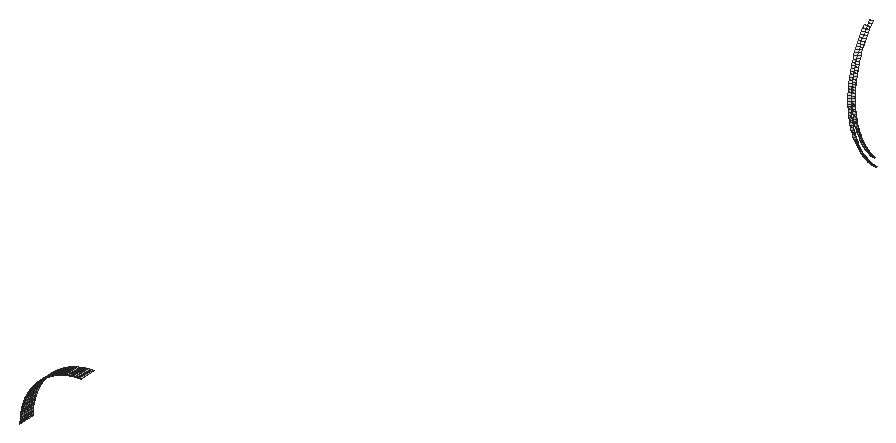
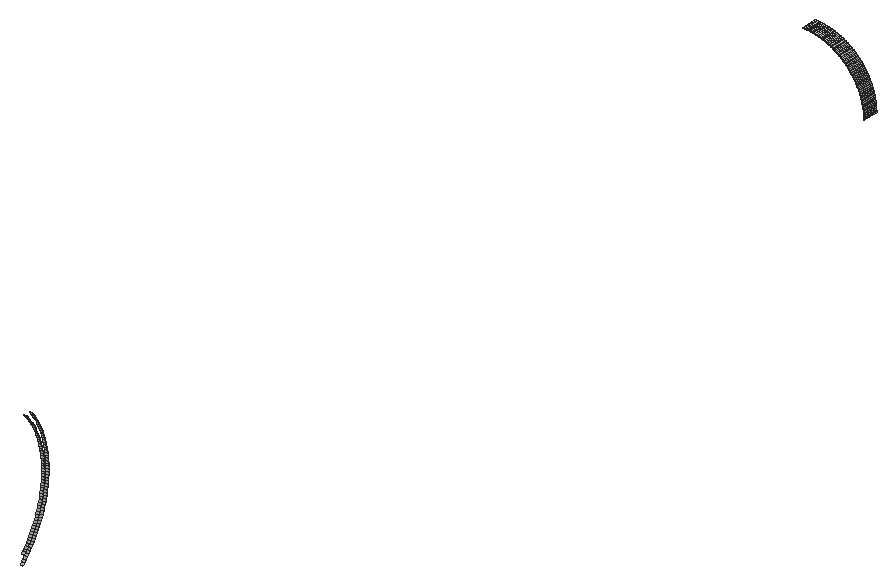
# SketchUp Ruby script. Lengths in inches.
U = 1.inch
M = Sketchup.active_model
def pt(a) = Geom::Point3d.new(a.map { |v| v * U })
def face(e, loops, mat)
  f = e.add_face(loops[0].map { |a| pt(a) })
  loops[1..].each { |l| e.add_face(l.map { |a| pt(a) }).erase! }
  f.material = f.back_material = mat if mat
  f
end
# faces: each face lists its corners as indices into pts; further lists are holes
def faces(e, pts, list, mat = nil) = list.each { |f| face(e, (f[0].is_a?(Array) ? f : [f]).map { |l| l.map { |i| pts[i] } }, mat) }
# xy, xz, yz: faces in a plane at the given z, y or x. An outline is a flat list of corners, or four numbers for a rectangle; further outlines are holes
def ring(l) = l.size == 4 ? [[l[0], l[1]], [l[2], l[1]], [l[2], l[3]], [l[0], l[3]]] : l.each_slice(2).to_a
def flat(e, list, mat, &to3) = list.each { |f| face(e, (f[0].is_a?(Array) ? f : [f]).map { |l| ring(l).map { |u, v| to3.(u, v) } }, mat) }
def xy(e, z, list, mat = nil) = flat(e, list, mat) { |x, y| [x, y, z] }
def xz(e, y, list, mat = nil) = flat(e, list, mat) { |x, z| [x, y, z] }
def yz(e, x, list, mat = nil) = flat(e, list, mat) { |y, z| [x, y, z] }
def lines(e, pts, list) = list.each { |a, b| e.add_line(pt(pts[a]), pt(pts[b])) }
# prism: a flat outline (further loops are holes) pulled along v
def prism(e, loops, v, mat = nil)
  f = face(e, loops, mat); d = Geom::Vector3d.new(v.map { |x| x * U })
  f.pushpull(f.normal.samedirection?(d) ? d.length : -d.length)
end
def box(e, o, s, mat = nil) = prism(e, [[o, [o[0] + s[0], o[1], o[2]], [o[0] + s[0], o[1] + s[1], o[2]], [o[0], o[1] + s[1], o[2]]]], [0, 0, s[2]], mat)
def at(x, y, z, deg = 0) = Geom::Transformation.translation(pt([x, y, z])) * Geom::Transformation.rotation(ORIGIN, Z_AXIS, deg.degrees)
def axes(o, x, y, z) = Geom::Transformation.new([*x, 0, *y, 0, *z, 0, *pt(o).to_a, 1])
def part(name) = M.definitions.add(name)
# library, detail: a bought-in or finely detailed component or shape, given as its bounding box
def library(name, o, s) = part(name).tap { |d| box(d.entities, o, s) }
def detail(e, o, s) = box(e.add_group.entities, o, s)
def put(e, d, t, mat = nil) = e.add_instance(d, t).tap { |i| i.material = mat if mat }
def group(e, t, mat = nil) = e.add_group.tap { |g| g.transformation = t; g.material = mat if mat }.entities
root = M.entities
M.materials.add("[Quartz Light Grey]").color = [251, 251, 252]
xy(root,66,[[23.6875,50,23.84,53],[23.84,50,24,53]])
xz(root,211,[[44.5,50.56,45,51.0625]],"[Quartz Light Grey]")
xz(root,212,[[44.5,50.59,45,51.06]],"[Quartz Light Grey]")
yz(root,12,[[50,54,53,54.16],[50,54.16,53,54.3125]])
p = [[45,216.875,37.26],[45,217.24,36.92],[44.5,217.24,36.92],[44.5,216.875,37.26],[45,216.52,37.61],[44.5,216.52,37.61],
  [45,216.18,37.97],[44.5,216.18,37.97],[45,215.84,38.33],[44.5,215.84,38.33],[45,215.51,38.71],[44.5,215.51,38.71],
  [45,215.2,39.09],[44.5,215.2,39.09],[45,216.9,38.65],[45,216.58,39],[44.5,216.58,39],[44.5,216.9,38.65],
  [45,216.27,39.35],[44.5,216.27,39.35],[45,214.89,39.48],[44.5,214.89,39.48],[45,215.97,39.72],[44.5,215.97,39.72],
  [45,214.59,39.88],[44.5,214.59,39.88],[45,215.68,40.09],[44.5,215.68,40.09],[45,214.31,40.29],[44.5,214.31,40.29],
  [45,215.4,40.47],[44.5,215.4,40.47],[45,214.03,40.7],[44.5,214.03,40.7],[45,215.13,40.85],[44.5,215.13,40.85],
  [45,213.77,41.125],[44.5,213.77,41.125],[45,214.87,41.25],[44.5,214.87,41.25],[45,213.51,41.55],[44.5,213.51,41.55],
  [45,214.62,41.65],[44.5,214.62,41.65],[45,213.27,41.99],[44.5,213.27,41.99],[45,214.38,42.05],[44.5,214.38,42.05],
  [45,213.04,42.43],[44.5,213.04,42.43],[45,214.15,42.46],[44.5,214.15,42.46],[45,212.82,42.875],[44.5,212.82,42.875],
  [45,213.94,42.88],[44.5,213.94,42.88],[45,212.62,43.33],[44.5,212.62,43.33],[45,213.73,43.3],[44.5,213.73,43.3],
  [45,212.42,43.79],[44.5,212.42,43.79],[45,213.53,43.73],[44.5,213.53,43.73],[45,213.35,44.17],[44.5,213.35,44.17],
  [45,212.24,44.25],[44.5,212.24,44.25],[45,212.07,44.72],[44.5,212.07,44.72],[45,213.17,44.6],[44.5,213.17,44.6],
  [45,213.01,45.05],[44.5,213.01,45.05],[45,211.91,45.1875],[44.5,211.91,45.1875],[45,212.86,45.49],[44.5,212.86,45.49],
  [45,211.76,45.66],[44.5,211.76,45.66],[45,212.72,45.94],[44.5,212.72,45.94],[45,211.63,46.14],[44.5,211.63,46.14],
  [45,212.6,46.4],[44.5,212.6,46.4],[45,211.51,46.625],[44.5,211.51,46.625],[45,212.48,46.86],[44.5,212.48,46.86],
  [45,211.4,47.11],[44.5,211.4,47.11],[45,212.38,47.31],[44.5,212.38,47.31],[45,211.31,47.6],[44.5,211.31,47.6],
  [45,212.29,47.78],[44.5,212.29,47.78],[45,211.22,48.09],[44.5,211.22,48.09],[45,212.21,48.24],[44.5,212.21,48.24],
  [45,211.15,48.58],[44.5,211.15,48.58],[45,212.15,48.71],[44.5,212.15,48.71],[45,211.1,49.08],[44.5,211.1,49.08],
  [45,212.09,49.18],[44.5,212.09,49.18],[45,211.05,49.57],[44.5,211.05,49.57],[45,212.05,49.65],[44.5,212.05,49.65],
  [45,211.02,50.07],[44.5,211.02,50.07],[45,212.02,50.12],[44.5,212.02,50.12],[45,211,50.56],[44.5,211,50.56],
  [45,212,50.59],[44.5,212,50.59],[45,211.01,51.56],[45,211,51.0625],[44.5,211,51.0625],[44.5,211.01,51.56],
  [45,212,51.06],[45,212.01,51.53],[44.5,212.01,51.53],[44.5,212,51.06],[45,212.03,52],[44.5,212.03,52],
  [45,211.03,52.06],[44.5,211.03,52.06],[45,212.06,52.47],[44.5,212.06,52.47],[45,211.0625,52.55],[44.5,211.0625,52.55],
  [45,212.1,52.94],[44.5,212.1,52.94],[45,211.11,53.05],[44.5,211.11,53.05],[45,212.16,53.41],[44.5,212.16,53.41],
  [45,211.17,53.54],[44.5,211.17,53.54],[45,212.23,53.875],[44.5,212.23,53.875],[45,211.24,54.03],[44.5,211.24,54.03],
  [45,212.3125,54.34],[44.5,212.3125,54.34],[45,211.33,54.52],[44.5,211.33,54.52],[12,53,54.3125],[12.01,53,54.47],
  [12.01,50,54.47],[12,50,54.3125],[45,212.41,54.8],[44.5,212.41,54.8],[12.02,53,54.63],[12.02,50,54.63],
  [45,211.43,55.01],[44.5,211.43,55.01],[12.03,53,54.78],[12.03,50,54.78],[12.04,53,54.94],[12.04,50,54.94],
  [45,212.51,55.26],[44.5,212.51,55.26],[12.05,53,55.1],[12.05,50,55.1],[45,211.54,55.5],[44.5,211.54,55.5],
  [12.07,53,55.25],[12.07,50,55.25],[12.08,53,55.41],[12.08,50,55.41],[45,212.63,55.72],[44.5,212.63,55.72],
  [12.1,53,55.57],[12.1,50,55.57],[45,211.66,55.98],[44.5,211.66,55.98],[12.125,53,55.72],[12.125,50,55.72],
  [12.15,53,55.88],[12.15,50,55.88],[45,212.76,56.17],[44.5,212.76,56.17],[12.17,53,56.03],[12.17,50,56.03],
  [12.2,53,56.1875],[12.2,50,56.1875],[45,211.8,56.46],[44.5,211.8,56.46],[12.23,53,56.34],[12.23,50,56.34],
  [45,212.9,56.62],[44.5,212.9,56.62],[12.26,53,56.49],[12.26,50,56.49],[12.3,53,56.65],[12.3,50,56.65],
  [45,211.95,56.93],[44.5,211.95,56.93],[12.33,53,56.8],[12.33,50,56.8],[45,213.05,57.0625],[44.5,213.05,57.0625],
  [12.37,53,56.95],[12.37,50,56.95],[45,212.11,57.4],[44.5,212.11,57.4],[12.41,53,57.11],[12.41,50,57.11],
  [12.45,53,57.26],[12.45,50,57.26],[45,213.22,57.51],[44.5,213.22,57.51],[12.49,53,57.41],[12.49,50,57.41],
  [12.54,53,57.56],[12.54,50,57.56],[45,212.28,57.87],[44.5,212.28,57.87],[45,213.39,57.94],[44.5,213.39,57.94],
  [12.59,53,57.71],[12.59,50,57.71],[12.64,53,57.86],[12.64,50,57.86],[12.6875,53,58.01],[12.6875,50,58.01],
  [45,212.47,58.33],[44.5,212.47,58.33],[45,213.58,58.375],[44.5,213.58,58.375],[12.74,53,58.15],[12.74,50,58.15],
  [12.8,53,58.3],[12.8,50,58.3],[12.85,53,58.45],[12.85,50,58.45],[45,212.67,58.78],[44.5,212.67,58.78],
  [12.91,53,58.59],[12.91,50,58.59],[45,213.78,58.8],[44.5,213.78,58.8],[12.97,53,58.74],[12.97,50,58.74],
  [13.04,53,58.88],[13.04,50,58.88],[45,212.88,59.24],[44.5,212.88,59.24],[45,213.99,59.22],[44.5,213.99,59.22],
  [13.1,53,59.02],[13.1,50,59.02],[13.17,53,59.17],[13.17,50,59.17],[13.24,53,59.31],[13.24,50,59.31],
  [45,213.1,59.68],[44.5,213.1,59.68],[45,214.21,59.64],[44.5,214.21,59.64],[13.31,53,59.45],[13.31,50,59.45],
  [13.38,53,59.59],[13.38,50,59.59],[13.45,53,59.73],[13.45,50,59.73],[45,214.44,60.05],[44.5,214.44,60.05],
  [13.53,53,59.86],[13.53,50,59.86],[45,213.33,60.12],[44.5,213.33,60.12],[13.61,53,60],[13.61,50,60],
  [13.6875,53,60.14],[13.6875,50,60.14],[13.77,53,60.27],[13.77,50,60.27],[45,213.58,60.55],[44.5,213.58,60.55],
  [45,214.68,60.45],[44.5,214.68,60.45],[13.85,53,60.4],[13.85,50,60.4],[13.9375,53,60.54],[13.9375,50,60.54],
  [14.02,53,60.67],[14.02,50,60.67],[45,214.9375,60.85],[44.5,214.9375,60.85],[45,213.83,60.98],[44.5,213.83,60.98],
  [14.11,53,60.8],[14.11,50,60.8],[14.2,53,60.93],[14.2,50,60.93],[14.29,53,61.05],[14.29,50,61.05],
  [45,215.2,61.24],[44.5,215.2,61.24],[45,214.1,61.4],[44.5,214.1,61.4],[14.38,53,61.18],[14.38,50,61.18],
  [14.48,53,61.31],[14.48,50,61.31],[45,215.47,61.63],[44.5,215.47,61.63],[14.58,53,61.43],[14.58,50,61.43],
  [14.67,53,61.55],[14.67,50,61.55],[45,214.375,61.8125],[44.5,214.375,61.8125],[14.77,53,61.67],[14.77,50,61.67],
  [45,215.76,62],[44.5,215.76,62],[14.875,53,61.79],[14.875,50,61.79],[14.98,53,61.91],[14.98,50,61.91],
  [45,214.67,62.22],[44.5,214.67,62.22],[15.08,53,62.03],[15.08,50,62.03],[15.1875,53,62.15],[15.1875,50,62.15],
  [45,216.05,62.375],[44.5,216.05,62.375],[15.3,53,62.26],[15.3,50,62.26],[45,214.96,62.62],[44.5,214.96,62.62],
  [15.4,53,62.375],[15.4,50,62.375],[15.51,53,62.49],[15.51,50,62.49],[45,216.35,62.73],[44.5,216.35,62.73],
  [15.625,53,62.6],[15.625,50,62.6],[15.74,53,62.7],[15.74,50,62.7],[15.85,53,62.8125],[15.85,50,62.8125],
  [15.97,53,62.92],[15.97,50,62.92],[16.09,53,63.02],[16.09,50,63.02],[16.21,53,63.125],[16.21,50,63.125],
  [16.33,53,63.23],[16.33,50,63.23],[16.45,53,63.33],[16.45,50,63.33],[16.57,53,63.42],[16.57,50,63.42],
  [16.69,53,63.52],[16.69,50,63.52],[16.82,53,63.62],[16.82,50,63.62],[16.95,53,63.71],[16.95,50,63.71],
  [17.07,53,63.8],[17.07,50,63.8],[17.2,53,63.89],[17.2,50,63.89],[17.33,53,63.98],[17.33,50,63.98],
  [17.46,53,64.0625],[17.46,50,64.0625],[17.6,53,64.15],[17.6,50,64.15],[17.73,53,64.23],[17.73,50,64.23],
  [17.86,53,64.3125],[17.86,50,64.3125],[18,53,64.39],[18,50,64.39],[18.14,53,64.47],[18.14,50,64.47],
  [18.27,53,64.55],[18.27,50,64.55],[18.41,53,64.62],[18.41,50,64.62],[18.55,53,64.69],[18.55,50,64.69],
  [18.69,53,64.76],[18.69,50,64.76],[18.83,53,64.83],[18.83,50,64.83],[18.98,53,64.9],[18.98,50,64.9],
  [19.12,53,64.96],[19.12,50,64.96],[19.26,53,65.03],[19.26,50,65.03],[19.41,53,65.09],[19.41,50,65.09],
  [19.55,53,65.15],[19.55,50,65.15],[19.7,53,65.2],[19.7,50,65.2],[19.85,53,65.26],[19.85,50,65.26],
  [19.99,53,65.3125],[19.99,50,65.3125],[20.14,53,65.36],[20.14,50,65.36],[20.29,53,65.41],[20.29,50,65.41],
  [20.44,53,65.46],[20.44,50,65.46],[20.59,53,65.51],[20.59,50,65.51],[20.74,53,65.55],[20.74,50,65.55],
  [20.89,53,65.59],[20.89,50,65.59],[21.05,53,65.63],[21.05,50,65.63],[21.2,53,65.67],[21.2,50,65.67],
  [21.35,53,65.7],[21.35,50,65.7],[21.51,53,65.74],[21.51,50,65.74],[21.66,53,65.77],[21.66,50,65.77],
  [21.8125,53,65.8],[21.8125,50,65.8],[21.97,53,65.83],[21.97,50,65.83],[22.12,53,65.85],[22.12,50,65.85],
  [22.28,53,65.875],[22.28,50,65.875],[22.43,53,65.9],[22.43,50,65.9],[22.59,53,65.92],[22.59,50,65.92],
  [22.75,53,65.93],[22.75,50,65.93],[22.9,53,65.95],[22.9,50,65.95],[23.06,53,65.96],[23.06,50,65.96],
  [23.22,53,65.97],[23.22,50,65.97],[23.37,53,65.98],[23.37,50,65.98],[23.53,53,65.99],[23.53,50,65.99],
  [23.6875,53,66],[23.6875,50,66]]
faces(root,p,[[0,1,2,3],[4,0,3,5],[6,4,5,7],[8,6,7,9],[10,8,9,11],[12,10,11,13],[14,15,16,17],[15,18,19,16],
  [20,12,13,21],[18,22,23,19],[24,20,21,25],[22,26,27,23],[28,24,25,29],[26,30,31,27],[32,28,29,33],[30,34,35,31],
  [36,32,33,37],[34,38,39,35],[40,36,37,41],[38,42,43,39],[44,40,41,45],[42,46,47,43],[48,44,45,49],[46,50,51,47],
  [52,48,49,53],[50,54,55,51],[56,52,53,57],[54,58,59,55],[60,56,57,61],[58,62,63,59],[62,64,65,63],[66,60,61,67],
  [68,66,67,69],[64,70,71,65],[70,72,73,71],[74,68,69,75],[72,76,77,73],[78,74,75,79],[76,80,81,77],[82,78,79,83],
  [80,84,85,81],[86,82,83,87],[84,88,89,85],[90,86,87,91],[88,92,93,89],[94,90,91,95],[92,96,97,93],[98,94,95,99],
  [96,100,101,97],[102,98,99,103],[100,104,105,101],[106,102,103,107],[104,108,109,105],[110,106,107,111],[108,112,113,109],[114,110,111,115],
  [112,116,117,113],[118,114,115,119],[116,120,121,117],[122,123,124,125],[126,127,128,129],[127,130,131,128],[132,122,125,133],[130,134,135,131],
  [136,132,133,137],[134,138,139,135],[140,136,137,141],[138,142,143,139],[144,140,141,145],[142,146,147,143],[148,144,145,149],[146,150,151,147],
  [152,148,149,153],[150,158,159,151],[162,152,153,163],[158,168,169,159],[172,162,163,173],[168,178,179,169],[182,172,173,183],[178,188,189,179],
  [194,182,183,195],[188,198,199,189],[204,194,195,205],[198,208,209,199],[212,204,205,213],[208,218,219,209],[224,212,213,225],[218,226,227,219],
  [234,224,225,235],[226,236,237,227],[244,234,235,245],[236,248,249,237],[254,244,245,255],[248,256,257,249],[264,254,255,265],[256,266,267,257],
  [266,274,275,267],[278,264,265,279],[286,278,279,287],[274,288,289,275],[288,296,297,289],[298,286,287,299],[296,306,307,297],[308,298,299,309],
  [306,314,315,307],[320,308,309,321],[314,324,325,315],[330,320,321,331],[324,336,337,325],[340,330,331,341],[336,346,347,337]],"[Quartz Light Grey]")
faces(root,p,[[154,155,156,157],[155,160,161,156],[160,164,165,161],[164,166,167,165],[166,170,171,167],[170,174,175,171],[174,176,177,175],[176,180,181,177],
  [180,184,185,181],[184,186,187,185],[186,190,191,187],[190,192,193,191],[192,196,197,193],[196,200,201,197],[200,202,203,201],[202,206,207,203],
  [206,210,211,207],[210,214,215,211],[214,216,217,215],[216,220,221,217],[220,222,223,221],[222,228,229,223],[228,230,231,229],[230,232,233,231],
  [232,238,239,233],[238,240,241,239],[240,242,243,241],[242,246,247,243],[246,250,251,247],[250,252,253,251],[252,258,259,253],[258,260,261,259],
  [260,262,263,261],[262,268,269,263],[268,270,271,269],[270,272,273,271],[272,276,277,273],[276,280,281,277],[280,282,283,281],[282,284,285,283],
  [284,290,291,285],[290,292,293,291],[292,294,295,293],[294,300,301,295],[300,302,303,301],[302,304,305,303],[304,310,311,305],[310,312,313,311],
  [312,316,317,313],[316,318,319,317],[318,322,323,319],[322,326,327,323],[326,328,329,327],[328,332,333,329],[332,334,335,333],[334,338,339,335],
  [338,342,343,339],[342,344,345,343],[344,348,349,345],[348,350,351,349],[350,352,353,351],[352,354,355,353],[354,356,357,355],[356,358,359,357],
  [358,360,361,359],[360,362,363,361],[362,364,365,363],[364,366,367,365],[366,368,369,367],[368,370,371,369],[370,372,373,371],[372,374,375,373],
  [374,376,377,375],[376,378,379,377],[378,380,381,379],[380,382,383,381],[382,384,385,383],[384,386,387,385],[386,388,389,387],[388,390,391,389],
  [390,392,393,391],[392,394,395,393],[394,396,397,395],[396,398,399,397],[398,400,401,399],[400,402,403,401],[402,404,405,403],[404,406,407,405],
  [406,408,409,407],[408,410,411,409],[410,412,413,411],[412,414,415,413],[414,416,417,415],[416,418,419,417],[418,420,421,419],[420,422,423,421],
  [422,424,425,423],[424,426,427,425],[426,428,429,427],[428,430,431,429],[430,432,433,431],[432,434,435,433],[434,436,437,435],[436,438,439,437],
  [438,440,441,439],[440,442,443,441],[442,444,445,443],[444,446,447,445],[446,448,449,447],[448,450,451,449],[450,452,453,451],[452,454,455,453],
  [454,456,457,455],[456,458,459,457],[458,460,461,459],[460,462,463,461]])
